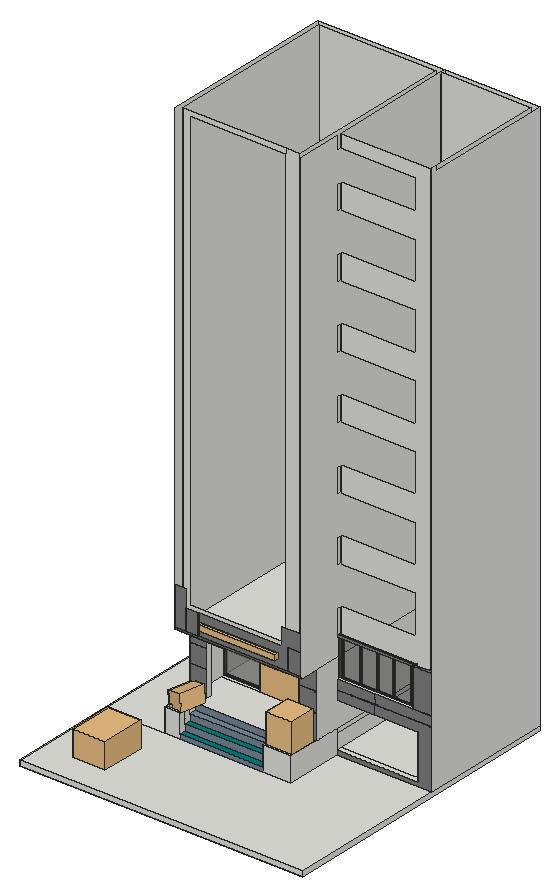
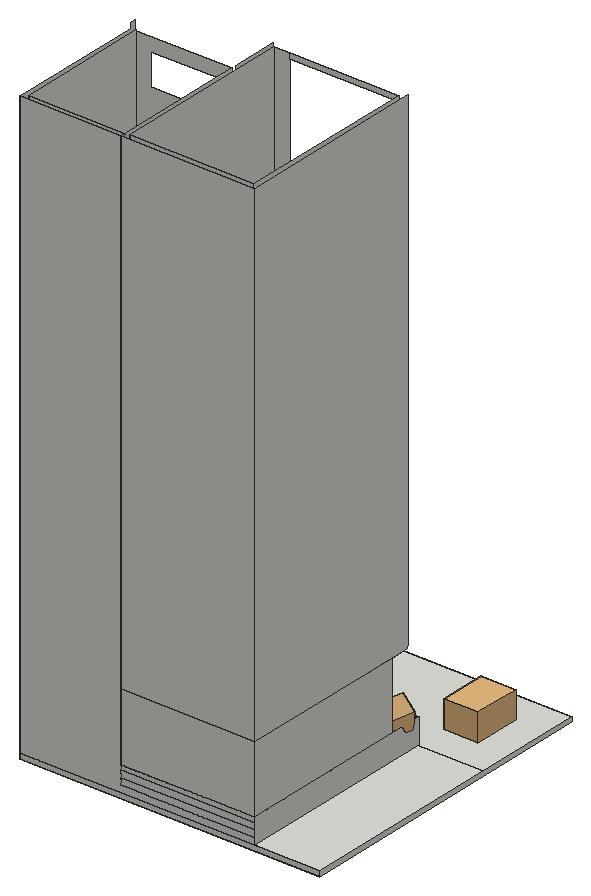
# SketchUp Ruby script. Lengths in inches.
U = 1.inch
M = Sketchup.active_model
def pt(a) = Geom::Point3d.new(a.map { |v| v * U })
def face(e, loops, mat)
  f = e.add_face(loops[0].map { |a| pt(a) })
  loops[1..].each { |l| e.add_face(l.map { |a| pt(a) }).erase! }
  f.material = f.back_material = mat if mat
  f
end
# faces: each face lists its corners as indices into pts; further lists are holes
def faces(e, pts, list, mat = nil) = list.each { |f| face(e, (f[0].is_a?(Array) ? f : [f]).map { |l| l.map { |i| pts[i] } }, mat) }
# xy, xz, yz: faces in a plane at the given z, y or x. An outline is a flat list of corners, or four numbers for a rectangle; further outlines are holes
def ring(l) = l.size == 4 ? [[l[0], l[1]], [l[2], l[1]], [l[2], l[3]], [l[0], l[3]]] : l.each_slice(2).to_a
def flat(e, list, mat, &to3) = list.each { |f| face(e, (f[0].is_a?(Array) ? f : [f]).map { |l| ring(l).map { |u, v| to3.(u, v) } }, mat) }
def xy(e, z, list, mat = nil) = flat(e, list, mat) { |x, y| [x, y, z] }
def xz(e, y, list, mat = nil) = flat(e, list, mat) { |x, z| [x, y, z] }
def yz(e, x, list, mat = nil) = flat(e, list, mat) { |y, z| [x, y, z] }
def lines(e, pts, list) = list.each { |a, b| e.add_line(pt(pts[a]), pt(pts[b])) }
# prism: a flat outline (further loops are holes) pulled along v
def prism(e, loops, v, mat = nil)
  f = face(e, loops, mat); d = Geom::Vector3d.new(v.map { |x| x * U })
  f.pushpull(f.normal.samedirection?(d) ? d.length : -d.length)
end
def box(e, o, s, mat = nil) = prism(e, [[o, [o[0] + s[0], o[1], o[2]], [o[0] + s[0], o[1] + s[1], o[2]], [o[0], o[1] + s[1], o[2]]]], [0, 0, s[2]], mat)
def at(x, y, z, deg = 0) = Geom::Transformation.translation(pt([x, y, z])) * Geom::Transformation.rotation(ORIGIN, Z_AXIS, deg.degrees)
def axes(o, x, y, z) = Geom::Transformation.new([*x, 0, *y, 0, *z, 0, *pt(o).to_a, 1])
def part(name) = M.definitions.add(name)
# library, detail: a bought-in or finely detailed component or shape, given as its bounding box
def library(name, o, s) = part(name).tap { |d| box(d.entities, o, s) }
def detail(e, o, s) = box(e.add_group.entities, o, s)
def put(e, d, t, mat = nil) = e.add_instance(d, t).tap { |i| i.material = mat if mat }
def group(e, t, mat = nil) = e.add_group.tap { |g| g.transformation = t; g.material = mat if mat }.entities
root = M.entities
M.materials.add("Aluminum_Anodized_DarkGray").color = [87, 83, 78]
M.materials.add("Glass_Coated_Black").color = [65, 65, 65]
M.materials["Glass_Coated_Black"].alpha = 0.42
M.materials.add("Material__1").color = [190, 136, 85]
M.materials.add("Material__2").color = [51, 42, 44]
M.materials.add("Material__3").color = [119, 136, 107]
M.materials.add("[0079_Teal]").color = [0, 128, 128]
M.materials.add("[0110_LightSlateGray]").color = [119, 136, 153]
M.materials.add("[0133_Gray]").color = [128, 128, 128]
M.materials.add("[0134_DimGray]").color = [105, 105, 105]
M.materials.add("[0137_Black]").color = [0, 0, 0]
M.materials.add("[Color M06]").color = [76, 76, 76]
M.materials.add("[Translucent Glass Gray]").color = [128, 128, 128]
M.materials["[Translucent Glass Gray]"].alpha = 0.5
c1 = library("2016+Honda+Civic+LX+Sedan",[0.01,0.03,0.02],[16.17,34.46,10.62])
c2 = library("Potted plant",[-35.72,-28.42,0],[66.31,67.39,78.4375])
c3 = library("\#2",[-119.83,-119.83,113.8],[239.66,239.66,17.4])
c4 = library("\#4",[-204.92,-212.35,-236.71],[424.28,257.5,472.53])
c5 = part("\#3")
put(c5.entities,c4,axes([-0.37,309.72,0],[1.36765,0,0],[0,1.36765,0],[0,0,1.36765]),"Material__3")
c6 = library("\#1",[-174.07,-174.07,0],[348.14,348.14,140])
c7 = part("9")
put(c7.entities,c3,at(-19.94,-24.66,0),"Material__2")
put(c7.entities,c5,axes([17.67,-32.6,40.29],[0.29694,0.9549,0],[-0.21403,0.06656,0.97456],[0.9306,-0.28939,0.22414]))
put(c7.entities,c6,at(-19.94,-24.66,0),"Material__1")
c8 = library("Group\#91",[-38.42,0,0],[76.84,15.04,96.4])
c9 = part("Group\#71")
box(c9.entities,[0,0,0],[0.5,123.75,116])
c10 = part("Group\#78")
xy(c10.entities,0,[[0,9.59,4.5,53.59]],"[Color M06]")
xy(c10.entities,2,[[0,9.59,4.5,11.59],[0,11.59,4.5,51.59]],"[Color M06]")
xy(c10.entities,118,[[0,9.59,4.5,11.59],[0,11.59,4.5,12.59],[0,12.59,4.5,51.59]],"[Color M06]")
xy(c10.entities,120,[[0,9.59,4.5,53.59]],"[Color M06]")
xz(c10.entities,9.59,[[0,0,4.5,2],[0,2,4.5,96],[0,96,4.5,98],[0,98,4.5,118],[0,118,4.5,120]],"[Color M06]")
xz(c10.entities,11.59,[[0,2,4.5,118]],"[Color M06]")
xz(c10.entities,51.59,[[0,2,4.5,118]],"[Color M06]")
xz(c10.entities,53.59,[[0,0,4.5,120]],"[Color M06]")
yz(c10.entities,0,[[9.59,0,9.59,2,51.59,2,51.59,118,9.59,118,9.59,120,53.59,120,53.59,0],[9.59,2,11.59,118]],"[Color M06]")
yz(c10.entities,4.5,[[9.59,0,53.59,0,53.59,120,9.59,120,9.59,118,51.59,118,51.59,2,9.59,2],[9.59,2,11.59,118]],"[Color M06]")
p = [[2,10.57,117.59],[2,10.57,98]]
lines(c10.entities,p,[[0,1]])
put(c10.entities,c9,axes([2.25,10.59,2],[1,0,0],[0,0.33131,0],[0,0,1]),"[Translucent Glass Gray]")
c11 = part("glass wall")
put(c11.entities,c8,at(9.7,25.35,0,90))
put(c11.entities,c10,axes([0,47.95,0],[1,0,0],[0,1.64948,0],[0,0,0.8]),"[Translucent Glass Gray]")
g1 = group(c11.entities,at(0,-85.65,0))
xy(g1,0,[[0,0,4.5,72.58]],"[Color M06]")
xy(g1,1.6,[[0,3.04,4.5,69.54],[0,69.54,4.5,71.06],[4.5,69.54,5.8125,71.06],[0,71.06,4.5,72.58],[4.5,71.06,5.8125,72.58]],"[Color M06]")
xy(g1,94.4,[[0,3.04,4.5,69.54],[0,69.54,4.5,71.06],[4.5,69.54,5.8125,71.06],[0,71.06,4.5,72.58],[4.5,71.06,5.8125,72.58]],"[Color M06]")
xy(g1,96,[[0,0,4.5,72.58]],"[Color M06]")
xz(g1,0,[[0,0,4.5,96]],"[Color M06]")
xz(g1,3.04,[[0,1.6,4.5,94.4]],"[Color M06]")
xz(g1,69.54,[[0,1.6,5.8125,94.4]],"[Color M06]")
xz(g1,72.58,[[0,0,4.5,1.6],[0,1.6,5.8125,76.8],[0,76.8,4.5,78.4],[4.5,76.8,5.8125,78.4],[0,78.4,5.8125,94.4],
  [0,94.4,4.5,96]],"[Color M06]")
yz(g1,0,[[0,0,0,96,72.58,96,72.58,94.4,3.04,94.4,3.04,1.6,72.58,1.6,72.58,0],[69.54,1.6,71.06,94.4],[71.06,1.6,72.58,94.4]],"[Color M06]")
yz(g1,4.5,[[0,0,72.58,0,72.58,1.6,3.04,1.6,3.04,94.4,72.58,94.4,72.58,96,0,96]],"[Color M06]")
yz(g1,5.8125,[[69.54,1.6,72.58,94.4]],"[Color M06]")
p = [[5.5625,72.54,78.4],[1.71,71.98,78.4],[5.5625,72.54,94.07],[1.71,71.98,94.07]]
lines(g1,p,[[0,1],[2,3],[1,3]])
put(g1,c9,axes([0,3.43,1.6],[1,0,0],[0,0.53419,0],[0,0,0.8]),"[Translucent Glass Gray]")
put(c11.entities,c10,axes([0,92.15,96],[1,0,0],[0,0.82474,0],[0,0,0.2]),"[Translucent Glass Gray]")
put(c11.entities,c10,axes([0,55.86,96],[1,0,0],[0,0.82474,0],[0,0,0.2]),"[Translucent Glass Gray]")
put(c11.entities,c10,axes([0,-57.27,96],[1,0,0],[0,0.82474,0],[0,0,0.2]),"[Translucent Glass Gray]")
put(c11.entities,c10,axes([0,-93.5625,96],[1,0,0],[0,0.82474,0],[0,0,0.2]),"[Translucent Glass Gray]")
put(c11.entities,c10,axes([0,-21.45,96],[1,0,0],[0,0.87325,0],[0,0,0.2]),"[Translucent Glass Gray]")
put(c11.entities,c10,axes([0,16.97,96],[1,0,0],[0,0.87325,0],[0,0,0.2]),"[Translucent Glass Gray]")
c12 = part("Group\#2")
xy(c12.entities,0,[[0,0,54,3]],"Aluminum_Anodized_DarkGray")
xy(c12.entities,2,[[2.25,0,51.75,1],[2.25,2,51.75,3]],"Aluminum_Anodized_DarkGray")
xy(c12.entities,3,[[3.375,1,14.625,1.5],[15.75,1,26.4375,1.5],[27.5625,1,38.25,1.5],[39.375,1,50.625,1.5],[3.375,1.5,14.625,2],
  [15.75,1.5,26.4375,2],[27.5625,1.5,38.25,2],[39.375,1.5,50.625,2]],"Aluminum_Anodized_DarkGray")
xy(c12.entities,99,[[3.375,1,14.625,1.5],[15.75,1,26.4375,1.5],[26.4375,1,27.5625,2],[27.5625,1,38.25,1.5],[38.25,1,39.375,2],
  [39.375,1,50.625,1.5],[3.375,1.5,14.625,2],[15.75,1.5,26.4375,2],[27.5625,1.5,38.25,2],[39.375,1.5,50.625,2]],"Aluminum_Anodized_DarkGray")
xy(c12.entities,100,[[2.25,0,51.75,1],[2.25,2,51.75,3]],"Aluminum_Anodized_DarkGray")
xy(c12.entities,102,[[0,0,54,3]],"Aluminum_Anodized_DarkGray")
xz(c12.entities,0,[[[0,0,54,102],[2.25,2,51.75,100]]],"Aluminum_Anodized_DarkGray")
xz(c12.entities,1,[[[2.25,2,51.75,100],[39.375,3,50.625,99],[3.375,3,14.625,99],[27.5625,3,38.25,99],[15.75,3,26.4375,99]]],"Aluminum_Anodized_DarkGray")
xz(c12.entities,1.5,[[3.375,3,14.625,99],[15.75,3,27,99],[27.5625,3,38.8125,99],[39.375,3,50.625,99]],"Glass_Coated_Black")
xz(c12.entities,2,[[[2.25,2,51.75,100],[39.375,3,50.625,99],[3.375,3,14.625,99],[27.5625,3,38.25,99],[15.75,3,26.4375,99]]],"Aluminum_Anodized_DarkGray")
xz(c12.entities,3,[[[0,0,54,102],[2.25,2,51.75,100]]],"Aluminum_Anodized_DarkGray")
yz(c12.entities,0,[[0,0,3,102]],"Aluminum_Anodized_DarkGray")
yz(c12.entities,2.25,[[0,2,1,100],[2,2,3,100]],"Aluminum_Anodized_DarkGray")
yz(c12.entities,3.375,[[1,3,1.5,99],[1.5,3,2,99]],"Aluminum_Anodized_DarkGray")
yz(c12.entities,14.625,[[1,3,1.5,99],[1.5,3,2,99]],"Aluminum_Anodized_DarkGray")
yz(c12.entities,15.75,[[1,3,1.5,99],[1.5,3,2,99]],"Aluminum_Anodized_DarkGray")
yz(c12.entities,26.4375,[[1,3,2,99]],"Aluminum_Anodized_DarkGray")
yz(c12.entities,27.5625,[[1,3,1.5,99],[1.5,3,2,99]],"Aluminum_Anodized_DarkGray")
yz(c12.entities,38.25,[[1,3,2,99]],"Aluminum_Anodized_DarkGray")
yz(c12.entities,39.375,[[1,3,1.5,99],[1.5,3,2,99]],"Aluminum_Anodized_DarkGray")
yz(c12.entities,50.625,[[1,3,1.5,99],[1.5,3,2,99]],"Aluminum_Anodized_DarkGray")
yz(c12.entities,51.75,[[0,2,1,100],[2,2,3,100]],"Aluminum_Anodized_DarkGray")
yz(c12.entities,54,[[0,0,3,102]],"Aluminum_Anodized_DarkGray")
p = [[15.75,2,99],[14.625,2,99]]
lines(c12.entities,p,[[0,1]])
c13 = library("COMPANY NAME",[0.42,0,0],[95.72,9.9,1])
xy(root,-54,[[0,0,535.9375,561.3125]])
xy(root,-45,[[0,0,535.9375,0,535.9375,305.1875,355.9375,305.1875,355.9375,197.1875,0,197.1875],[0,197.1875,115.9375,561.3125],[115.9375,197.1875,355.9375,197.1875,355.9375,305.1875,535.9375,305.1875,535.9375,561.3125,115.9375,561.3125]])
xy(root,-36,[[355.9375,305.1875,510.375,314.1875],[355.9375,314.1875,526.9375,552.3125]])
xy(root,-36,[[144.4375,197.1875,302.625,209.1875]],"[0079_Teal]")
xy(root,-28.5,[[311.625,206.1875,346.9375,248.1875]])
xy(root,-24,[[144.4375,209.1875,302.625,221.1875]],"[0079_Teal]")
xy(root,-12,[[144.4375,221.1875,302.625,233.1875]],"[0110_LightSlateGray]")
xy(root,-11.75,[[119.9375,201.1875,140.4375,253.1875]])
xy(root,0,[[[115.9375,197.1875,144.4375,257.1875],[119.9375,201.1875,140.4375,253.1875]],[[302.625,197.1875,355.9375,257.1875],[311.625,206.1875,346.9375,248.1875]],[144.4375,233.1875,302.625,233.1875,302.625,257.1875,322.9375,257.1875,322.9375,266.1875,346.9375,266.1875,346.9375,321.3125,124.9375,321.3125,124.9375,266.1875,149.1875,266.1875,149.1875,257.1875,144.4375,257.1875],[115.9375,257.1875,124.9375,257.1875,124.9375,552.3125,346.9375,552.3125,346.9375,266.1875,322.9375,266.1875,322.9375,257.1875,355.9375,257.1875,355.9375,561.3125,115.9375,561.3125],[124.9375,257.1875,149.1875,266.1875],
  [124.9375,321.3125,346.9375,330.3125],[124.9375,330.3125,346.9375,552.3125]])
xy(root,47.5,[[115.9375,257.1875,149.1875,257.6875],[322.9375,257.1875,355.9375,257.6875]])
xy(root,48,[[115.9375,257.1875,149.1875,257.6875],[322.9375,257.1875,355.9375,257.6875],[355.9375,305.1875,510.375,314.1875]])
xy(root,83.5,[[115.9375,257.1875,149.1875,257.6875],[322.9375,257.1875,355.9375,257.6875]])
xy(root,84,[[115.9375,257.1875,149.1875,257.6875],[322.9375,257.1875,355.9375,257.6875],[355.9375,305.1875,499.9375,314.1875]])
xy(root,120,[[115.9375,223.1875,124.9375,257.1875],[124.9375,223.1875,160.9375,257.1875],[160.9375,223.1875,160.9375,257.1875,149.1875,257.1875,149.1875,266.1875,124.9375,266.1875,124.9375,552.3125,346.9375,552.3125,346.9375,266.1875,322.9375,266.1875,322.9375,257.1875,310.9375,257.1875,310.9375,223.1875],[310.9375,223.1875,346.9375,257.1875],[346.9375,223.1875,355.9375,257.1875],
  [115.9375,257.1875,115.9375,561.3125,355.9375,561.3125,355.9375,257.1875,346.9375,257.1875,346.9375,552.3125,124.9375,552.3125,124.9375,257.1875],[124.9375,257.1875,149.1875,266.1875],[322.9375,257.1875,346.9375,266.1875]])
xy(root,125,[[115.9375,221.1875,115.9375,223.1875,355.9375,223.1875,355.9375,221.1875,330.6875,221.1875,330.6875,221.6875,330.1875,221.6875,330.1875,221.1875,161.25,221.1875,161.25,221.6875,160.75,221.6875,160.75,221.1875,137.25,221.1875,137.25,221.6875,136.75,221.6875,136.75,221.1875]])
xy(root,129,[[124.9375,230.1875,346.9375,552.3125]])
xy(root,156,[[355.9375,305.1875,499.9375,314.1875]])
xz(root,0,[[0,-54,535.9375,-45]])
xz(root,197.1875,[[115.9375,-45,144.4375,0],[302.625,-45,355.9375,0]])
xz(root,197.1875,[[144.4375,-45,302.625,-36]],"[0110_LightSlateGray]")
xz(root,201.1875,[[119.9375,-11.75,140.4375,0]])
xz(root,206.1875,[[311.625,-28.5,346.9375,0]])
xz(root,209.1875,[[144.4375,-36,302.625,-24]],"[0110_LightSlateGray]")
xz(root,221.1875,[[144.4375,-24,302.625,-12]],"[0110_LightSlateGray]")
xz(root,221.1875,[[115.9375,125,136.75,125,136.75,165,136.9375,165,136.9375,197.24,115.9375,197.24],[137.25,125,160.75,165],[161.25,125,330.1875,125,330.1875,165.75,355.9375,165.75,355.9375,197.24,319.9375,197.24,319.9375,165,161.25,165],[330.6875,125,355.9375,165.25]],"[0133_Gray]")
xz(root,221.6875,[[136.75,125,137.25,165],[160.75,125,161.25,165],[330.1875,125,330.6875,125,330.6875,165.25,355.9375,165.25,355.9375,165.75,330.1875,165.75]],"[0137_Black]")
xz(root,223.1875,[[115.9375,120,355.9375,125]],"[0134_DimGray]")
xz(root,230.1875,[[124.9375,129,124.9375,1005,319.75,1005,319.75,996,136.9375,996,136.9375,165,319.9375,165,319.9375,129],[319.9375,129,346.9375,1005]])
xz(root,233.1875,[[144.4375,-12,302.625,0]],"[0110_LightSlateGray]")
xz(root,248.1875,[[311.625,-28.5,346.9375,0]])
xz(root,253.1875,[[119.9375,-11.75,140.4375,0]])
xz(root,257.1875,[[115.9375,0,149.1875,47.5],[322.9375,0,355.9375,47.5],[115.9375,48,149.1875,83.5],[322.9375,48,355.9375,83.5],[115.9375,84,149.1875,120],
  [322.9375,84,355.9375,120]],"[0133_Gray]")
xz(root,257.6875,[[115.9375,47.5,149.1875,48],[322.9375,47.5,355.9375,48],[115.9375,83.5,149.1875,84],[322.9375,83.5,355.9375,84]])
xz(root,266.1875,[[124.9375,0,149.1875,120],[322.9375,0,346.9375,120]])
xz(root,305.1875,[[427.65,48,428.15,65.5],[355.9375,65.5,427.65,66],[427.65,65.5,428.15,66],[428.15,65.5,535.9375,66],[427.65,66,428.15,84],
  [499.9375,83.5,535.9375,84]])
xz(root,305.1875,[[355.9375,-45,535.9375,-45,535.9375,65.5,428.15,65.5,428.15,48,510.375,48,510.375,-36,355.9375,-36],[355.9375,48,427.65,65.5],[355.9375,66,427.65,84],[428.15,66,535.9375,66,535.9375,83.5,499.9375,83.5,499.9375,84,428.15,84],[499.9375,84,535.9375,156],
  [355.9375,156,517.9375,160],[517.9375,156,535.9375,160]],"[0133_Gray]")
xz(root,314.1875,[[510.375,-36,510.375,48,355.9375,48,355.9375,84,499.9375,84,499.9375,156,355.9375,156,355.9375,204,499.37,204,499.37,276.01,355.9375,276.01,355.9375,324,499.37,324,499.37,396,355.9375,396,355.9375,444,499.37,444,499.37,516.13,355.9375,516.13,355.9375,564,499.37,564,499.37,636,355.9375,636,355.9375,684,499.37,684,499.37,756,355.9375,756,355.9375,804,499.37,804,499.37,876,355.9375,876,355.9375,924,499.37,924,499.37,981,355.9375,981,355.9375,1005,526.9375,1005,526.9375,-36]])
xz(root,552.3125,[[355.9375,-36,526.9375,1005],[124.9375,0,346.9375,120],[124.9375,129,346.9375,1005]])
xz(root,561.3125,[[0,-54,535.9375,-45],[115.9375,-45,115.9375,-33,355.9375,-33,355.9375,1005.1875,535.9375,1005.1875,535.9375,-45],[115.9375,-33,355.9375,-21],[115.9375,-21,355.9375,-9],[115.9375,-9,355.9375,0],
  [115.9375,0,355.9375,120],[115.9375,120,355.9375,1005]])
yz(root,0,[[0,-54,561.3125,-45]])
yz(root,115.9375,[[197.1875,-45,561.3125,0],[257.1875,0,257.1875,47.5,257.6875,47.5,257.6875,48,257.1875,48,257.1875,83.5,257.6875,83.5,257.6875,84,257.1875,84,257.1875,120,561.3125,120,561.3125,0],[223.1875,120,223.1875,125,221.1875,125,221.1875,197.24,221.6875,197.24,221.6875,197.74,221.1875,197.74,221.1875,230.48,221.6875,230.48,221.6875,230.98,221.1875,230.98,221.1875,263.72,221.6875,263.72,221.6875,264.22,221.1875,264.22,221.1875,297.46,221.6875,297.46,221.6875,297.96,221.1875,297.96,221.1875,330.2,221.6875,330.2,221.6875,330.7,221.1875,330.7,221.1875,363.94,221.6875,363.94,221.6875,364.44,221.1875,364.44,221.1875,397.18,221.6875,397.18,221.6875,397.68,221.1875,397.68,221.1875,430.42,221.6875,430.42,221.6875,430.88,221.1875,430.88,221.1875,463.16,221.6875,463.16,221.6875,463.66,221.1875,463.66,221.1875,496.4,221.6875,496.4,221.6875,496.9,221.1875,496.9,221.1875,530.14,221.6875,530.14,221.6875,530.64,221.1875,530.64,221.1875,562.88,221.6875,562.88,221.6875,563.38,221.1875,563.38,221.1875,596.12,221.6875,596.12,221.6875,596.62,221.1875,596.62,221.1875,629.36,221.6875,629.36,221.6875,629.86,221.1875,629.86,221.1875,663.1,221.6875,663.1,221.6875,663.6,221.1875,663.6,221.1875,696.34,221.6875,696.34,221.6875,696.84,221.1875,696.84,221.1875,729.08,221.6875,729.08,221.6875,729.58,221.1875,729.58,221.1875,762.82,221.6875,762.82,221.6875,763.32,221.1875,763.32,221.1875,796.04,221.6875,796.04,221.6875,796.56,221.1875,796.56,221.1875,828.8,221.6875,828.8,221.6875,829.3,221.1875,829.3,221.1875,862.04,221.6875,862.04,221.6875,862.54,221.1875,862.54,221.1875,895.28,221.6875,895.28,221.6875,895.78,221.1875,895.78,221.1875,928.52,221.6875,928.52,221.6875,929.02,221.1875,929.02,221.1875,961.76,221.6875,961.76,221.6875,962.26,221.1875,962.26,221.1875,1005,561.3125,1005,561.3125,120]])
yz(root,119.9375,[[201.1875,-11.75,253.1875,0]])
yz(root,124.9375,[[266.1875,0,552.3125,120],[230.1875,129,552.3125,1005]])
yz(root,136.75,[[221.1875,125,221.6875,165]])
yz(root,137.25,[[221.1875,125,221.6875,165]])
yz(root,140.4375,[[201.1875,-11.75,253.1875,0]])
yz(root,144.4375,[[197.1875,-36,209.1875,0],[209.1875,-24,221.1875,0],[221.1875,-12,233.1875,0]])
yz(root,149.1875,[[257.1875,0,266.1875,0,266.1875,120,257.1875,120,257.1875,84,257.6875,84,257.6875,83.5,257.1875,83.5,257.1875,48,257.6875,48,257.6875,47.5,257.1875,47.5]])
yz(root,160.75,[[221.1875,125,221.6875,165]])
yz(root,161.25,[[221.1875,125,221.6875,165]])
yz(root,302.625,[[197.1875,-36,209.1875,0],[209.1875,-24,221.1875,0],[221.1875,-12,233.1875,0]])
yz(root,311.625,[[206.1875,-28.5,248.1875,0]])
yz(root,322.9375,[[257.1875,0,257.1875,47.5,257.6875,47.5,257.6875,48,257.1875,48,257.1875,83.5,257.6875,83.5,257.6875,84,257.1875,84,257.1875,120,266.1875,120,266.1875,0]])
yz(root,330.1875,[[221.1875,125,221.6875,165.75]])
yz(root,330.6875,[[221.1875,125,221.6875,165.25]])
yz(root,346.9375,[[206.1875,-28.5,248.1875,0],[266.1875,0,552.3125,120],[230.1875,129,552.3125,1005]])
yz(root,355.9375,[[197.1875,-45,305.1875,0],[305.1875,-36,552.3125,-9],[305.1875,-9,552.3125,0],[[257.1875,0,552.3125,0,552.3125,120,257.1875,120,257.1875,84,257.6875,84,257.6875,83.5,257.1875,83.5,257.1875,48,257.6875,48,257.6875,47.5,257.1875,47.5],[305.1875,48,314.1875,84]],[552.3125,0,561.3125,120],
  [[223.1875,120,552.3125,120,552.3125,1005,314.1875,1005,314.1875,981,305.1875,981,305.1875,1005,221.1875,1005,221.1875,962.26,221.6875,962.26,221.6875,961.76,221.1875,961.76,221.1875,929.02,221.6875,929.02,221.6875,928.52,221.1875,928.52,221.1875,895.78,221.6875,895.78,221.6875,895.28,221.1875,895.28,221.1875,862.54,221.6875,862.54,221.6875,862.04,221.1875,862.04,221.1875,829.3,221.6875,829.3,221.6875,828.8,221.1875,828.8,221.1875,796.56,221.6875,796.56,221.6875,796.06,221.1875,796.06,221.1875,763.32,221.6875,763.32,221.6875,762.82,221.1875,762.82,221.1875,729.58,221.6875,729.58,221.6875,729.08,221.1875,729.08,221.1875,696.84,221.6875,696.84,221.6875,696.34,221.1875,696.34,221.1875,663.6,221.6875,663.6,221.6875,663.1,221.1875,663.1,221.1875,629.86,221.6875,629.86,221.6875,629.36,221.1875,629.36,221.1875,596.62,221.6875,596.62,221.6875,596.12,221.1875,596.12,221.1875,563.38,221.6875,563.38,221.6875,562.88,221.1875,562.88,221.1875,530.64,221.75,530.64,221.75,530.14,221.1875,530.14,221.1875,496.9,221.25,496.9,221.25,496.4,221.1875,496.4,221.1875,463.66,221.3125,463.66,221.3125,463.16,221.1875,463.16,221.1875,430.92,221.3125,430.92,221.3125,430.42,221.1875,430.42,221.1875,397.68,221.6875,397.68,221.6875,397.18,221.1875,397.18,221.1875,364.44,221.6875,364.44,221.6875,363.94,221.1875,363.94,221.1875,330.7,221.6875,330.7,221.6875,330.2,221.1875,330.2,221.1875,297.96,221.6875,297.96,221.6875,297.46,221.1875,297.46,221.1875,264.22,221.6875,264.22,221.6875,263.72,221.1875,263.72,221.1875,230.98,221.6875,230.98,221.6875,230.48,221.1875,230.48,221.1875,197.74,221.6875,197.74,221.6875,197.24,221.1875,197.24,221.1875,165.75,221.6875,165.75,221.6875,165.25,221.1875,165.25,221.1875,125,223.1875,125],[305.1875,756,314.1875,804],[305.1875,156,314.1875,204],[305.1875,396,314.1875,444],[305.1875,636,314.1875,684],[305.1875,876,314.1875,924],[305.1875,276.01,314.1875,324],[305.1875,516.13,314.1875,564]],[552.3125,120,561.3125,1005]])
yz(root,499.9375,[[305.1875,84,314.1875,156]])
yz(root,510.375,[[305.1875,-36,314.1875,48]])
yz(root,526.9375,[[314.1875,-36,552.3125,1005.1875]])
yz(root,535.9375,[[0,-54,561.3125,-45],[305.1875,-45,561.3125,-45,561.3125,1005.1875,552.3125,1005.1875,552.3125,1005,314.1875,1005,314.1875,1014,305.1875,1014]])
put(root,c1,axes([55.98,55.8,-45.1],[3.772,0,0],[0,2.4178,0],[0,0,4.5489]))
put(root,c2,axes([330.1875,224.25,-28.5],[0.73,0,0],[0,0.75,0],[0,0,1.0688]))
put(root,c7,axes([134.125,229.77,-12],[0.056,0,0],[0,0.083,0],[0,0,0.09067]))
put(root,c11,at(210.59,330.3125,0,-90))
put(root,c12,axes([355.9375,311.1875,84],[2.66667,0,0],[0,0.5,0],[0,0,0.71]))
put(root,c13,axes([165.91,221.1875,139.07],[1.51305,0,0],[0,0,1],[0,-6.45,0]))
